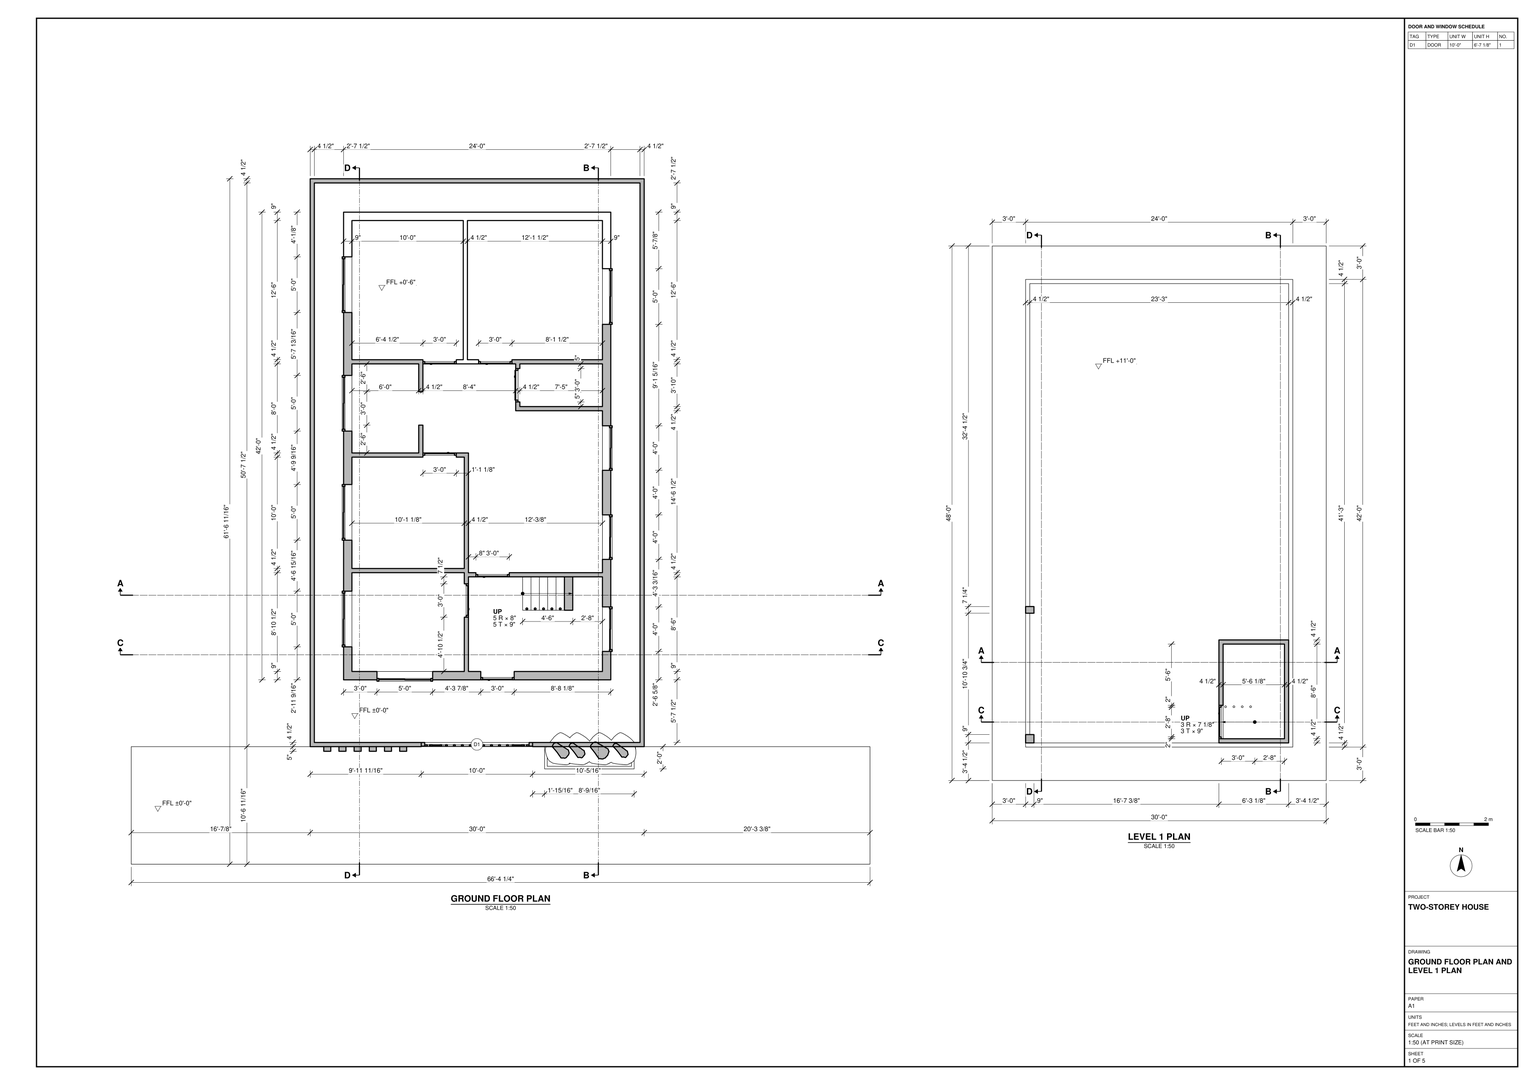
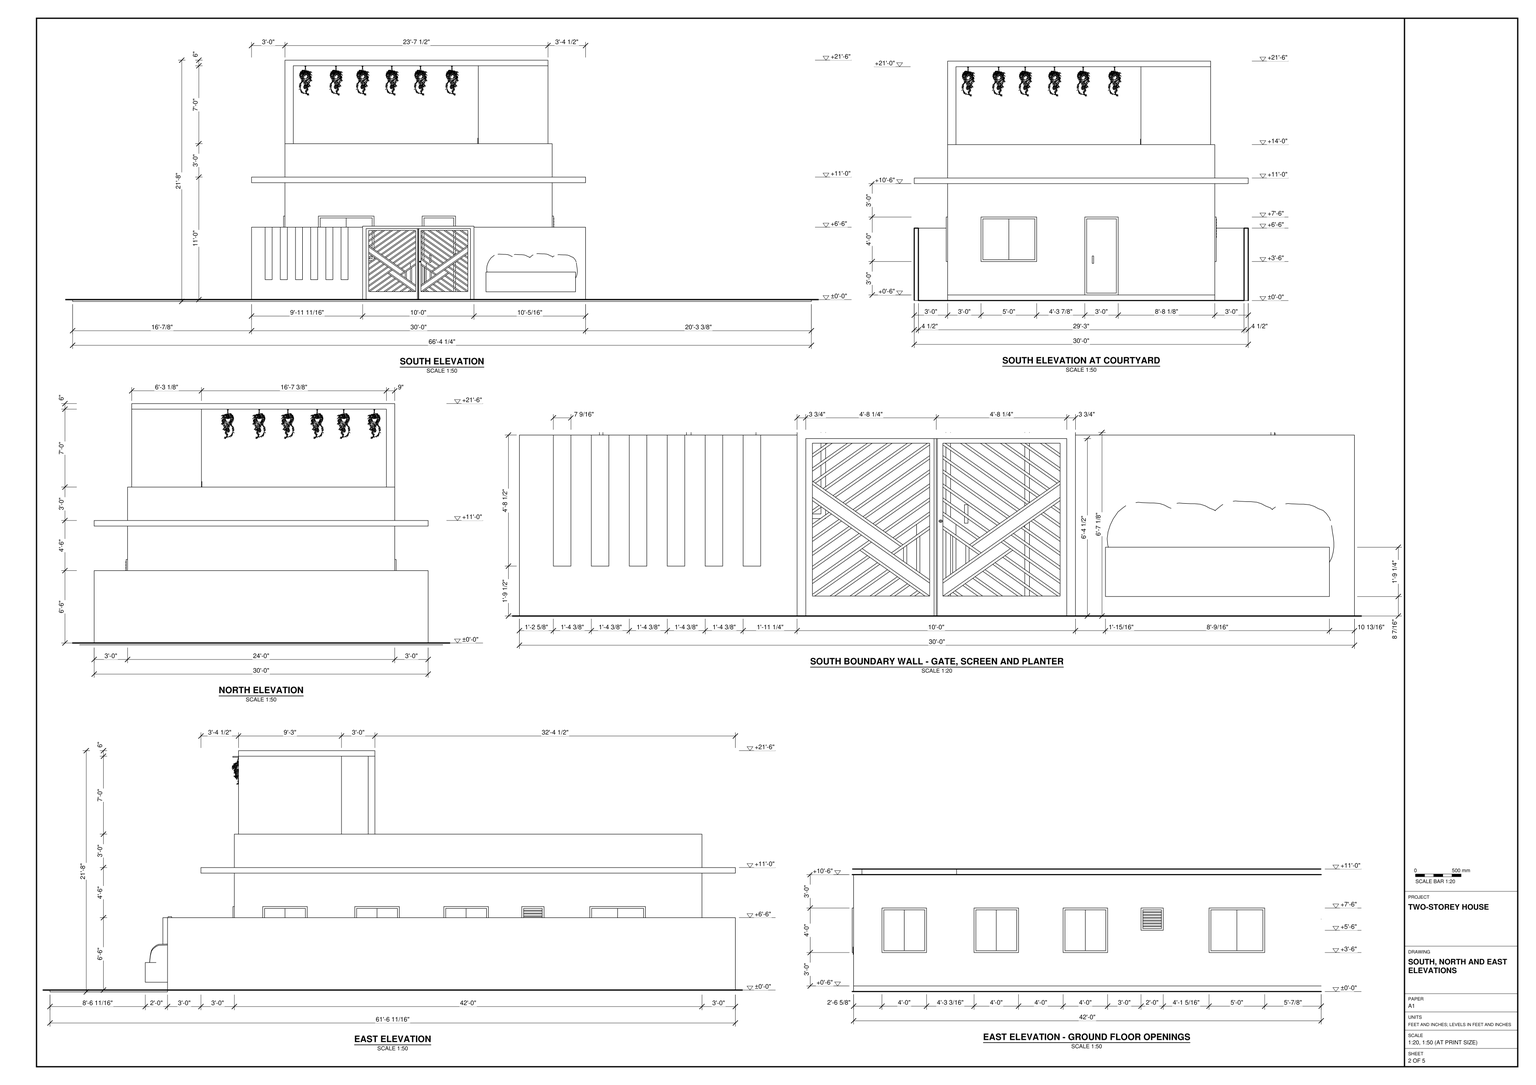
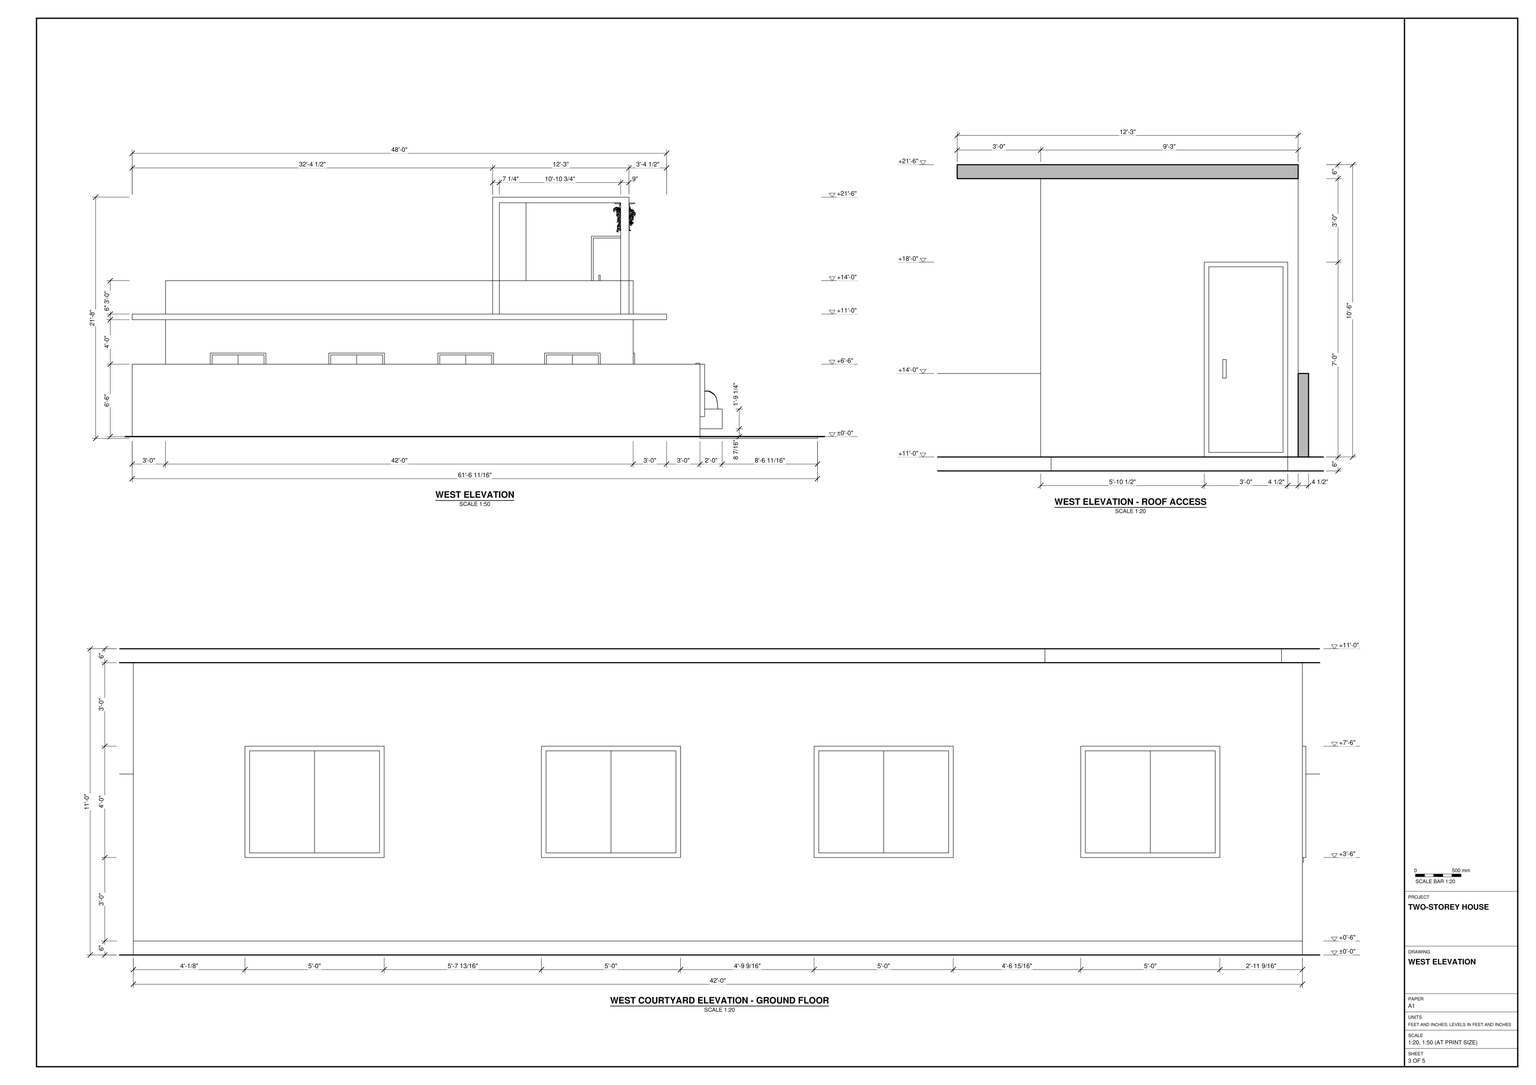
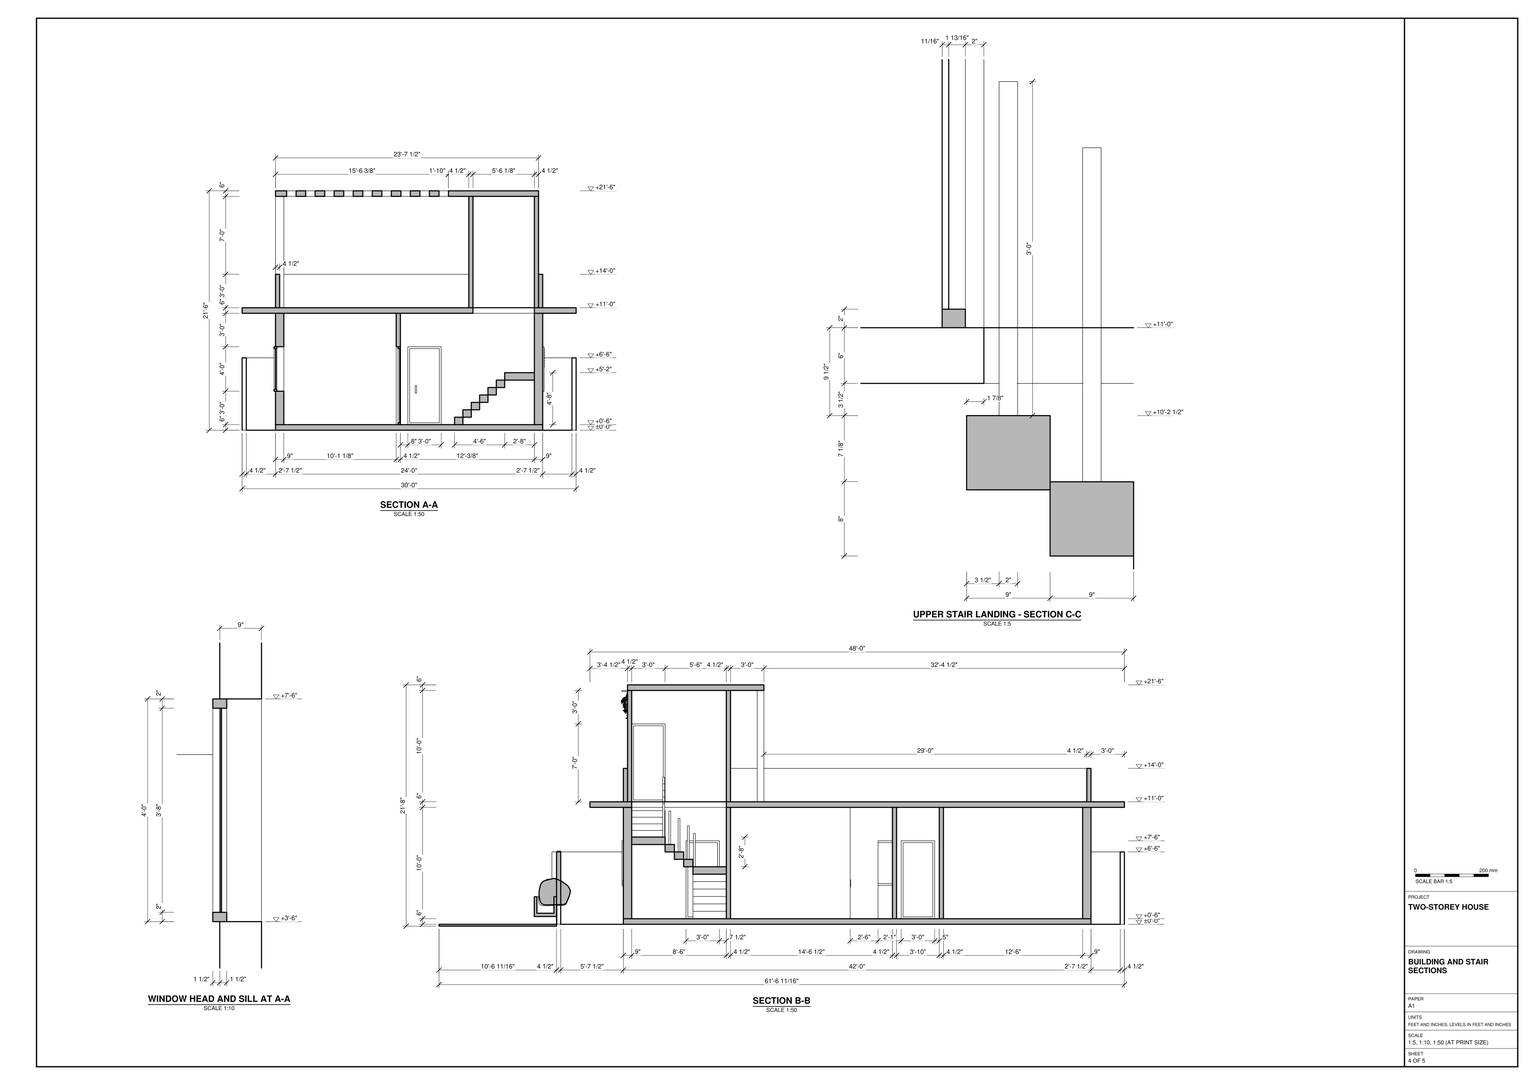
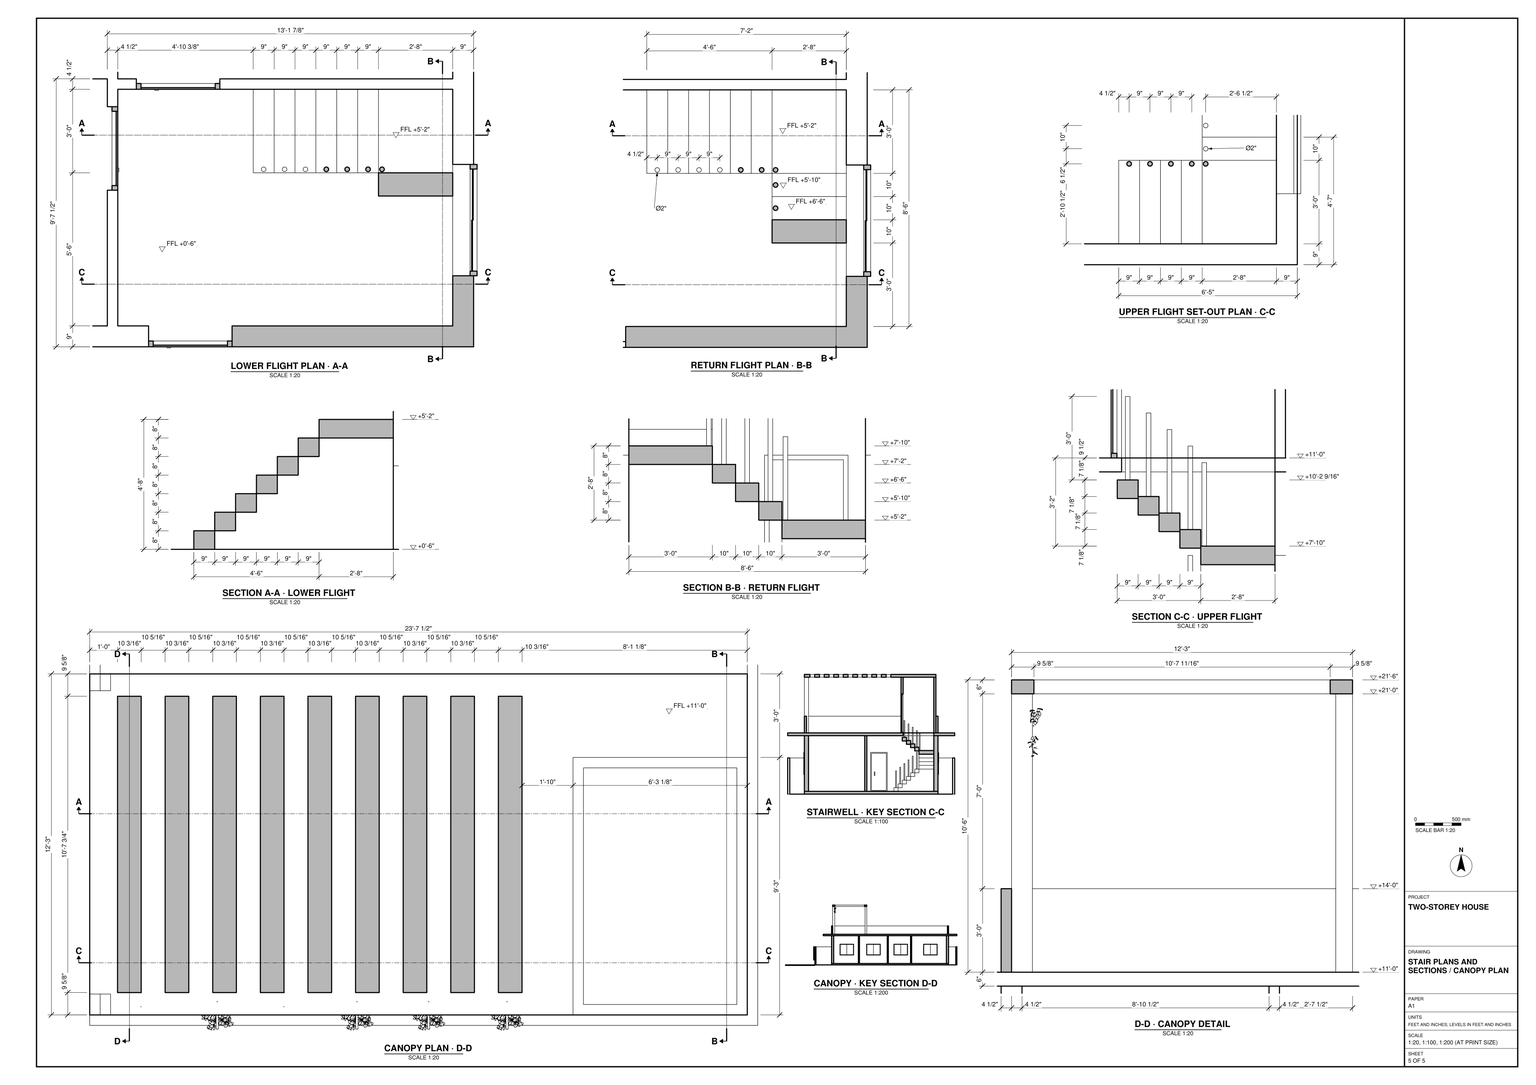
Build the house and its enclosed courtyard in SketchUp using task_files/diagram_01.pdf. Work in feet and inches. Including the ground strip outside the south boundary, the overall model extents are 66'-4 1/4" east to west, 61'-6 11/16" north to south and 21'-8" vertically. Use ±0'-0" as the ground datum and +11'-0" as the roof terrace level. Set the interior ground floor at +0'-6" as shown.

Lay out the rectangular house inside the boundary walls. Use 9" exterior walls and 4 1/2" interior partitions, following the room divisions and doorway positions on the ground floor plan. Model the courtyard entrance, window units and east wall vent from the elevations. At the south boundary, place the double gate between the slotted screen and the projecting planter.

Build the floor slabs and the stair at the southeast end of the house. Show how the stair reaches the roof access enclosure and opens onto the terrace. Distinguish the projecting terrace slab, the parapet set back from its edge and the higher flat roof over the access area. Decor and loose items, including the plants at the planter and beneath the upper roof, may be any suitable library components.

Keep walls, slabs, stairs and roofs in separate groups or components, and do the same for each furniture or joinery piece shown. Use components for repeated parts. Save one SketchUp model as output_files/two_storey_house_with_a_courtyard_and_roof_terrace.skp.

# SketchUp Ruby script. Lengths in inches.
U = 1.inch
M = Sketchup.active_model
def pt(a) = Geom::Point3d.new(a.map { |v| v * U })
def face(e, loops, mat)
  f = e.add_face(loops[0].map { |a| pt(a) })
  loops[1..].each { |l| e.add_face(l.map { |a| pt(a) }).erase! }
  f.material = f.back_material = mat if mat
  f
end
# faces: each face lists its corners as indices into pts; further lists are holes
def faces(e, pts, list, mat = nil) = list.each { |f| face(e, (f[0].is_a?(Array) ? f : [f]).map { |l| l.map { |i| pts[i] } }, mat) }
# xy, xz, yz: faces in a plane at the given z, y or x. An outline is a flat list of corners, or four numbers for a rectangle; further outlines are holes
def ring(l) = l.size == 4 ? [[l[0], l[1]], [l[2], l[1]], [l[2], l[3]], [l[0], l[3]]] : l.each_slice(2).to_a
def flat(e, list, mat, &to3) = list.each { |f| face(e, (f[0].is_a?(Array) ? f : [f]).map { |l| ring(l).map { |u, v| to3.(u, v) } }, mat) }
def xy(e, z, list, mat = nil) = flat(e, list, mat) { |x, y| [x, y, z] }
def xz(e, y, list, mat = nil) = flat(e, list, mat) { |x, z| [x, y, z] }
def yz(e, x, list, mat = nil) = flat(e, list, mat) { |y, z| [x, y, z] }
def lines(e, pts, list) = list.each { |a, b| e.add_line(pt(pts[a]), pt(pts[b])) }
# prism: a flat outline (further loops are holes) pulled along v
def prism(e, loops, v, mat = nil)
  f = face(e, loops, mat); d = Geom::Vector3d.new(v.map { |x| x * U })
  f.pushpull(f.normal.samedirection?(d) ? d.length : -d.length)
end
def box(e, o, s, mat = nil) = prism(e, [[o, [o[0] + s[0], o[1], o[2]], [o[0] + s[0], o[1] + s[1], o[2]], [o[0], o[1] + s[1], o[2]]]], [0, 0, s[2]], mat)
def at(x, y, z, deg = 0) = Geom::Transformation.translation(pt([x, y, z])) * Geom::Transformation.rotation(ORIGIN, Z_AXIS, deg.degrees)
def axes(o, x, y, z) = Geom::Transformation.new([*x, 0, *y, 0, *z, 0, *pt(o).to_a, 1])
def part(name) = M.definitions.add(name)
# library, detail: a bought-in or finely detailed component or shape, given as its bounding box
def library(name, o, s) = part(name).tap { |d| box(d.entities, o, s) }
def detail(e, o, s) = box(e.add_group.entities, o, s)
def put(e, d, t, mat = nil) = e.add_instance(d, t).tap { |i| i.material = mat if mat }
def group(e, t, mat = nil) = e.add_group.tap { |g| g.transformation = t; g.material = mat if mat }.entities
root = M.entities
M.materials.add("Asphalt A02 100cm").color = [81, 81, 83]
M.materials.add("Cementine Hexagonal Tiles 255cm").color = [92, 92, 95]
M.materials.add("Flooring Parquet Parallel E01 120cm").color = [119, 88, 63]
M.materials.add("Glass Clear 001").color = [0, 0, 0]
M.materials["Glass Clear 001"].alpha = 0.1
M.materials.add("Marble Emperador Dark 150cm").color = [81, 67, 62]
M.materials.add("Marble White SSS 100cm").color = [222, 222, 222]
M.materials.add("Metal Sandblasted Black 200cm").color = [86, 90, 95]
M.materials.add("Porcelain A02 Orange 10cm").color = [209, 126, 69]
M.materials.add("Porcelain C01 20cm").color = [125, 165, 163]
M.materials.add("Two Color Maple Panels 300cm").color = [56, 46, 41]
M.materials.add("Venetian Plaster Shadow 300cm").color = [61, 58, 77]
c1 = library("Skimmia japonica Rubella 004",[-17.08,-16.64,-0.26],[33.2,34.59,28.81])
c2 = library("Hanging Plant 111-02",[-6.97,-7.06,-31.95],[13.94,14.12,31.95])
c3 = library("gate 175k",[0,0,0],[125.98,4.13,118.11])
c4 = part("Group\#3")
box(c4.entities,[0,0,0],[28,0.31,44])
c5 = part("Group\#5")
box(c5.entities,[0,0,0],[0.31,28,44])
c6 = part("Group\#7")
box(c6.entities,[0,0,0],[0.31,28,44])
c7 = part("Group\#9")
box(c7.entities,[0,0,0],[0.31,28,44])
c8 = part("Group\#11")
box(c8.entities,[0,0,0],[0.31,28,44])
c9 = part("Group\#13")
box(c9.entities,[-0.31,0,0],[0.31,28,44])
c10 = library("Group\#14",[-1.5,0,0],[3.31,24,24])
c11 = part("Group\#17")
box(c11.entities,[-0.31,0,0],[0.31,22,44])
c12 = part("Group\#19")
box(c12.entities,[-0.31,0,0],[0.31,22,44])
c13 = part("Group\#21")
box(c13.entities,[-0.31,0,0],[0.31,22,44])
c14 = library("Group\#46",[0,0,0],[9,36,44])
c15 = library("Group\#49",[0,0,0],[9,36,44])
c16 = library("Group\#51",[0,0,0],[9,36,44])
c17 = library("Group\#53",[0,0,0],[9,36,44])
c18 = library("Group\#55",[0,0,0],[9,36,44])
c19 = library("Group\#57",[0,0,0],[9,36,44])
c20 = library("Group\#45",[0,0,0],[32,36,44])
c21 = library("Group\#48",[0,0,0],[32,10,44])
c22 = library("Group\#62",[0,0,0],[32,10,44])
c23 = library("Group\#64",[0,-2.5,0],[32,12.5,52])
c24 = library("Group\#59",[0,0,0],[9,36,44])
c25 = library("Group\#68",[0,0,0],[9,36,44])
c26 = library("Group\#70",[0,0,0],[9,36,44])
c27 = library("Group\#72",[0,0,0],[9,36,44])
c28 = library("Group\#75",[-0.5,0,0],[75.64,111,120])
put(root,c1,at(463.34,123.86,14.48))
put(root,c1,at(480.94,123.86,14.16))
put(root,c1,at(505.1875,123.86,15.05))
put(root,c1,at(527.875,123.86,13.94))
put(root,c2,at(251.0625,212.83,246))
put(root,c2,at(284.01,203.1875,246))
put(root,c2,at(312.64,212.83,246))
put(root,c2,at(344.21,203.1875,246))
put(root,c2,at(375.125,203.1875,246))
put(root,c2,at(408.96,203.1875,246))
put(root,c3,axes([312.59,127.05,-6],[0.9525,0,0],[0,1,0],[0,0,0.67]))
g1 = group(root,at(228.875,198.6875,0))
xy(g1,0,[[0,0,0,504,288,504,288,0,183.875,0,183.875,9,279,9,279,111,178.6,111,178.6,115.5,279,115.5,279,290,185.5,290,185.5,299.5,190,299.5,190,294.5,279,294.5,279,340.5,190,340.5,190,335.5,185.5,335.5,185.5,340.5,181.5,340.5,181.5,345,279,345,279,495,133.5,495,133.5,345,145.5,345,145.5,340.5,121.5,340.5,121.5,345,129,345,129,495,9,495,9,345,85.5,345,85.5,310.5,81,310.5,81,340.5,9,340.5,9,244.5,81,244.5,81,274.5,85.5,274.5,85.5,240,9,240,9,120,130.1,120,130.1,240,121.5,240,121.5,244.5,134.6,244.5,134.6,115.5,142.6,115.5,142.6,111,134.6,111,134.6,103.5,130.1,103.5,130.1,115.5,9,115.5,9,9,130.1,9,130.1,67.5,134.6,67.5,134.6,9,147.875,9,147.875,0]],"Venetian Plaster Shadow 300cm")
xy(g1,36,[[36,0,96,9],[279,30.61,288,78.61],[0,35.5625,9,95.5625],[279,129.8,288,177.8],[0,150.5,9,210.5],
  [279,225.8,288,273.8],[0,268.0625,9,328.0625],[279,383.11,288,443.11],[0,395.875,9,455.875]])
xy(g1,60,[[279,309.8,288,333.8]])
xy(g1,84,[[36,0,96,9],[147.875,0,183.875,9],[279,30.61,288,78.61],[0,35.5625,9,95.5625],[130.1,67.5,134.6,103.5],
  [142.6,111,178.6,115.5],[279,129.8,288,177.8],[0,150.5,9,210.5],[279,225.8,288,273.8],[85.5,240,121.5,244.5],
  [0,268.0625,9,328.0625],[81,274.5,85.5,310.5],[185.5,299.5,190,335.5],[279,309.8,288,333.8],[85.5,340.5,121.5,345],
  [145.5,340.5,181.5,345],[279,383.11,288,443.11],[0,395.875,9,455.875]])
xy(g1,120,[[[0,0,288,504],[134.6,115.5,134.6,244.5,85.5,244.5,85.5,340.5,185.5,340.5,185.5,290,279,290,279,115.5],[133.5,345,279,495],[9,345,129,495],[134.6,9,279,111],[9,120,130.1,240],[9,9,130.1,115.5],[9,244.5,81,340.5],[190,294.5,279,340.5]]])
xz(g1,0,[[[0,0,147.875,0,147.875,84,183.875,84,183.875,0,288,0,288,120,0,120],[36,36,96,84]]],"Porcelain C01 20cm")
xz(g1,9,[[[9,0,130.1,120],[36,36,96,84]],[134.6,0,134.6,120,279,120,279,0,183.875,0,183.875,84,147.875,84,147.875,0]],"Venetian Plaster Shadow 300cm")
xz(g1,30.61,[[279,36,288,84]])
xz(g1,35.5625,[[0,36,9,84]])
xz(g1,67.5,[[130.1,0,134.6,84]])
xz(g1,78.61,[[279,36,288,84]])
xz(g1,95.5625,[[0,36,9,84]])
xz(g1,103.5,[[130.1,0,134.6,84]])
xz(g1,111,[[134.6,0,142.6,0,142.6,84,178.6,84,178.6,0,279,0,279,120,134.6,120]],"Venetian Plaster Shadow 300cm")
xz(g1,115.5,[[9,0,130.1,120],[134.6,0,134.6,120,279,120,279,0,178.6,0,178.6,84,142.6,84,142.6,0]],"Venetian Plaster Shadow 300cm")
xz(g1,120,[[9,0,130.1,120]],"Venetian Plaster Shadow 300cm")
xz(g1,129.8,[[279,36,288,84]])
xz(g1,150.5,[[0,36,9,84]])
xz(g1,177.8,[[279,36,288,84]])
xz(g1,210.5,[[0,36,9,84]])
xz(g1,225.8,[[279,36,288,84]])
xz(g1,240,[[9,0,85.5,0,85.5,84,121.5,84,121.5,0,130.1,0,130.1,120,9,120]],"Venetian Plaster Shadow 300cm")
xz(g1,244.5,[[9,0,81,120],[121.5,0,121.5,84,85.5,84,85.5,120,134.6,120,134.6,0]],"Venetian Plaster Shadow 300cm")
xz(g1,268.0625,[[0,36,9,84]])
xz(g1,273.8,[[279,36,288,84]])
xz(g1,274.5,[[81,0,85.5,84]])
xz(g1,290,[[185.5,0,279,120]],"Venetian Plaster Shadow 300cm")
xz(g1,294.5,[[190,0,279,120]],"Venetian Plaster Shadow 300cm")
xz(g1,299.5,[[185.5,0,190,84]])
xz(g1,309.8,[[279,60,288,84]])
xz(g1,310.5,[[81,0,85.5,84]])
xz(g1,328.0625,[[0,36,9,84]])
xz(g1,333.8,[[279,60,288,84]])
xz(g1,335.5,[[185.5,0,190,84]])
xz(g1,340.5,[[9,0,81,120],[121.5,0,145.5,0,145.5,84,181.5,84,181.5,0,185.5,0,185.5,120,85.5,120,85.5,84,121.5,84],[190,0,279,120]],"Venetian Plaster Shadow 300cm")
xz(g1,345,[[9,0,9,120,129,120,129,0,121.5,0,121.5,84,85.5,84,85.5,0],[133.5,0,133.5,120,279,120,279,0,181.5,0,181.5,84,145.5,84,145.5,0]],"Venetian Plaster Shadow 300cm")
xz(g1,383.11,[[279,36,288,84]])
xz(g1,395.875,[[0,36,9,84]])
xz(g1,443.11,[[279,36,288,84]])
xz(g1,455.875,[[0,36,9,84]])
xz(g1,495,[[9,0,129,120],[133.5,0,279,120]],"Venetian Plaster Shadow 300cm")
xz(g1,504,[[0,0,288,120]],"Porcelain C01 20cm")
yz(g1,0,[[[0,0,504,120],[395.875,36,455.875,84],[268.0625,36,328.0625,84],[150.5,36,210.5,84],[35.5625,36,95.5625,84]]],"Porcelain C01 20cm")
yz(g1,9,[[[9,0,115.5,120],[35.5625,36,95.5625,84]],[[120,0,240,120],[150.5,36,210.5,84]],[[244.5,0,340.5,120],[268.0625,36,328.0625,84]],[[345,0,495,120],[395.875,36,455.875,84]]],"Venetian Plaster Shadow 300cm")
yz(g1,36,[[0,36,9,84]])
yz(g1,81,[[244.5,0,244.5,120,340.5,120,340.5,0,310.5,0,310.5,84,274.5,84,274.5,0]],"Venetian Plaster Shadow 300cm")
yz(g1,85.5,[[240,0,274.5,0,274.5,84,310.5,84,310.5,0,345,0,345,84,340.5,84,340.5,120,244.5,120,244.5,84,240,84]],"Venetian Plaster Shadow 300cm")
yz(g1,96,[[0,36,9,84]])
yz(g1,121.5,[[240,0,244.5,84],[340.5,0,345,84]])
yz(g1,129,[[345,0,495,120]],"Venetian Plaster Shadow 300cm")
yz(g1,130.1,[[9,0,9,120,115.5,120,115.5,0,103.5,0,103.5,84,67.5,84,67.5,0],[120,0,240,120]],"Venetian Plaster Shadow 300cm")
yz(g1,133.5,[[345,0,495,120]],"Venetian Plaster Shadow 300cm")
yz(g1,134.6,[[9,0,67.5,0,67.5,84,103.5,84,103.5,0,111,0,111,120,9,120],[115.5,0,244.5,120]],"Venetian Plaster Shadow 300cm")
yz(g1,142.6,[[111,0,115.5,84]])
yz(g1,145.5,[[340.5,0,345,84]])
yz(g1,147.875,[[0,0,9,84]])
yz(g1,178.6,[[111,0,115.5,84]])
yz(g1,181.5,[[340.5,0,345,84]])
yz(g1,183.875,[[0,0,9,84]])
yz(g1,185.5,[[290,0,290,120,340.5,120,340.5,0,335.5,0,335.5,84,299.5,84,299.5,0]],"Venetian Plaster Shadow 300cm")
yz(g1,190,[[294.5,0,299.5,0,299.5,84,335.5,84,335.5,0,340.5,0,340.5,120,294.5,120]],"Venetian Plaster Shadow 300cm")
yz(g1,279,[[[9,0,111,120],[30.61,36,78.61,84]]])
yz(g1,279,[[[115.5,0,290,120],[225.8,36,273.8,84],[129.8,36,177.8,84]],[[294.5,0,340.5,120],[309.8,60,333.8,84]],[[345,0,495,120],[383.11,36,443.11,84]]],"Venetian Plaster Shadow 300cm")
yz(g1,288,[[[0,0,504,120],[383.11,36,443.11,84],[225.8,36,273.8,84],[30.61,36,78.61,84],[129.8,36,177.8,84],[309.8,60,333.8,84]]],"Porcelain C01 20cm")
g2 = group(g1,at(36,0,36))
prism(g2,[[[0,-1.5,0],[60,-1.5,0],[60,-1.5,48],[0,-1.5,48]],[[58,-1.5,2],[2,-1.5,2],[2,-1.5,46],[58,-1.5,46]]],[0,3,0],"Metal Sandblasted Black 200cm")
put(g2,c4,at(2,0.25,2),"Glass Clear 001")
put(g2,c4,at(30,-0.06,2),"Glass Clear 001")
g3 = group(g1,at(0,35.5625,36))
prism(g3,[[[-1.5,0,0],[-1.5,0,48],[-1.5,60,48],[-1.5,60,0]],[[-1.5,2,2],[-1.5,58,2],[-1.5,58,46],[-1.5,2,46]]],[3,0,0],"Metal Sandblasted Black 200cm")
put(g3,c5,at(0.0625,30,2),"Glass Clear 001")
put(g3,c5,at(-0.25,2,2),"Glass Clear 001")
g4 = group(g1,at(0,150.5,36))
prism(g4,[[[-1.5,0,0],[-1.5,0,48],[-1.5,60,48],[-1.5,60,0]],[[-1.5,58,46],[-1.5,2,46],[-1.5,2,2],[-1.5,58,2]]],[3,0,0],"Metal Sandblasted Black 200cm")
put(g4,c6,at(0,30,2),"Glass Clear 001")
put(g4,c6,at(-0.31,2,2),"Glass Clear 001")
g5 = group(g1,at(0,268.0625,36))
prism(g5,[[[-1.5,60,0],[-1.5,0,0],[-1.5,0,48],[-1.5,60,48]],[[-1.5,2,46],[-1.5,2,2],[-1.5,58,2],[-1.5,58,46]]],[3,0,0],"Metal Sandblasted Black 200cm")
put(g5,c7,at(0.0625,30,2),"Glass Clear 001")
put(g5,c7,at(-0.25,2,2),"Glass Clear 001")
g6 = group(g1,at(0,395.875,36))
xy(g6,0,[[-1.5,0,1.5,60]])
xy(g6,2,[[-1.5,2,1.5,58]])
xy(g6,46,[[-1.5,2,1.5,58]])
xy(g6,48,[[-1.5,0,1.5,60]])
xz(g6,0,[[-1.5,0,1.5,48]])
xz(g6,2,[[-1.5,2,1.5,46]])
xz(g6,58,[[-1.5,2,1.5,46]])
xz(g6,60,[[-1.5,0,1.5,48]])
yz(g6,-1.5,[[[0,0,60,48],[2,2,58,46]]],"Metal Sandblasted Black 200cm")
yz(g6,1.5,[[[0,0,60,48],[2,2,58,46]]])
put(g6,c8,at(-0.1875,30,2),"Glass Clear 001")
put(g6,c8,at(-0.5,2,2),"Glass Clear 001")
g7 = group(g1,at(288,383.11,36))
prism(g7,[[[1.5,0,0],[1.5,60,0],[1.5,60,48],[1.5,0,48]],[[1.5,58,46],[1.5,58,2],[1.5,2,2],[1.5,2,46]]],[-3,0,0],"Metal Sandblasted Black 200cm")
put(g7,c9,at(-0.25,2,2),"Glass Clear 001")
put(g7,c9,at(0.06,30,2),"Glass Clear 001")
put(g1,c10,at(288,309.8,60))
g8 = group(g1,at(288,225.8,36))
prism(g8,[[[1.5,0,0],[1.5,48,0],[1.5,48,48],[1.5,0,48]],[[1.5,46,46],[1.5,46,2],[1.5,2,2],[1.5,2,46]]],[-3,0,0],"Metal Sandblasted Black 200cm")
put(g8,c11,at(0,2,2),"Glass Clear 001")
put(g8,c11,at(0.31,24,2),"Glass Clear 001")
g9 = group(g1,at(288,129.8,36))
prism(g9,[[[1.5,48,0],[1.5,48,48],[1.5,0,48],[1.5,0,0]],[[1.5,46,46],[1.5,46,2],[1.5,2,2],[1.5,2,46]]],[-3,0,0],"Metal Sandblasted Black 200cm")
put(g9,c12,at(-0.4375,2,2),"Glass Clear 001")
put(g9,c12,at(-0.12,24,2),"Glass Clear 001")
g10 = group(g1,at(288,30.61,36))
prism(g10,[[[1.5,48,0],[1.5,48,48],[1.5,0,48],[1.5,0,0]],[[1.5,46,46],[1.5,46,2],[1.5,2,2],[1.5,2,46]]],[-3,0,0],"Metal Sandblasted Black 200cm")
put(g10,c13,at(-0.5,2,2),"Glass Clear 001")
put(g10,c13,at(-0.19,24,2),"Glass Clear 001")
g11 = group(g1,at(147.875,0,0))
prism(g11,[[[36,0,0],[36,0,84],[0,0,84],[0,0,0]],[[34,0,82],[34,0,2],[2,0,2],[2,0,82]]],[0,2.5,0],"Metal Sandblasted Black 200cm")
g12 = group(g11,at(2,0,2))
box(g12,[0,0,0],[32,0.71,80],"Two Color Maple Panels 300cm")
g13 = group(g12,at(6,0,32),"Metal Sandblasted Black 200cm")
box(g13,[0,-0.5,0],[1.5,0.5,8])
g14 = group(g1,at(134.6,67.5,0))
prism(g14,[[[0,36,0],[0,36,84],[0,0,84],[0,0,0]],[[0,2,82],[0,34,82],[0,34,2],[0,2,2]]],[-2.5,0,0],"Metal Sandblasted Black 200cm")
g15 = group(g14,at(0,2,2))
xy(g15,0,[[-0.71,0,0,32]])
xy(g15,80,[[-0.71,0,0,32]])
xz(g15,0,[[-0.71,0,0,80]])
xz(g15,32,[[-0.71,0,0,80]])
yz(g15,-0.71,[[0,0,32,80]],"Two Color Maple Panels 300cm")
yz(g15,0,[[0,0,32,80]],"Two Color Maple Panels 300cm")
g16 = group(g15,at(0,6,32),"Metal Sandblasted Black 200cm")
box(g16,[0,0,0],[0.5,1.5,8])
g17 = group(g1,at(142.6,111,0))
prism(g17,[[[0,0,0],[36,0,0],[36,0,84],[0,0,84]],[[34,0,82],[34,0,2],[2,0,2],[2,0,82]]],[0,2.5,0],"Metal Sandblasted Black 200cm")
g18 = group(g17,at(2,0,2))
box(g18,[0,0,0],[32,0.71,80],"Two Color Maple Panels 300cm")
g19 = group(g18,at(6,0,32),"Metal Sandblasted Black 200cm")
box(g19,[0,-0.5,0],[1.5,0.5,8])
g20 = group(g1,at(145.5,340.5,0))
prism(g20,[[[0,0,0],[36,0,0],[36,0,84],[0,0,84]],[[2,0,82],[34,0,82],[34,0,2],[2,0,2]]],[0,2.5,0],"Metal Sandblasted Black 200cm")
g21 = group(g20,at(2,0,2))
box(g21,[0,0,0],[32,0.71,80],"Two Color Maple Panels 300cm")
g22 = group(g21,at(6,0,32),"Metal Sandblasted Black 200cm")
box(g22,[0,-0.5,0],[1.5,0.5,8])
g23 = group(g1,at(85.5,340.5,0))
prism(g23,[[[36,0,0],[36,0,84],[0,0,84],[0,0,0]],[[34,0,82],[34,0,2],[2,0,2],[2,0,82]]],[0,2.5,0],"Metal Sandblasted Black 200cm")
g24 = group(g23,at(2,0,2))
box(g24,[0,0,0],[32,0.71,80],"Two Color Maple Panels 300cm")
g25 = group(g24,at(6,0,32),"Metal Sandblasted Black 200cm")
box(g25,[0,-0.5,0],[1.5,0.5,8])
g26 = group(g1,at(185.5,299.5,0))
prism(g26,[[[0,0,0],[0,0,84],[0,36,84],[0,36,0]],[[0,2,82],[0,2,2],[0,34,2],[0,34,82]]],[2.5,0,0],"Metal Sandblasted Black 200cm")
g27 = group(g26,at(0,2,2))
box(g27,[-0.71,0,0],[0.71,32,80],"Two Color Maple Panels 300cm")
g28 = group(g27,at(-0.71,26,32),"Metal Sandblasted Black 200cm")
box(g28,[-0.5,-1.5,0],[0.5,1.5,8])
g29 = group(g1,at(85.5,244.5,0))
prism(g29,[[[36,0,84],[36,0,0],[0,0,0],[0,0,84]],[[2,0,82],[2,0,2],[34,0,2],[34,0,82]]],[0,-2.5,0],"Metal Sandblasted Black 200cm")
g30 = group(g29,at(2,0,2))
box(g30,[0,-0.71,0],[32,0.71,80],"Two Color Maple Panels 300cm")
g31 = group(g30,at(26,0,32),"Metal Sandblasted Black 200cm")
box(g31,[-1.5,0,0],[1.5,0.5,8])
g32 = group(root,at(228.875,198.6875,-6))
box(g32,[0,0,0],[288,504,6],"Marble White SSS 100cm")
put(root,c14,at(421.875,273.6875,0))
put(root,c15,at(430.875,273.6875,8))
put(root,c16,at(439.875,273.6875,16))
put(root,c17,at(448.875,273.6875,24))
put(root,c18,at(457.875,273.6875,32))
put(root,c19,at(466.875,273.6875,40))
put(root,c20,at(475.875,273.6875,48))
put(root,c21,at(475.875,263.6875,56))
put(root,c22,at(475.875,253.6875,64))
put(root,c23,at(475.875,243.6875,72))
g33 = group(root,at(475.875,233.6875,80))
box(g33,[0,-26,0],[32,36,8],"Marble White SSS 100cm")
put(root,c24,at(466.875,207.6875,87.13))
put(root,c25,at(457.875,207.6875,94.26))
put(root,c26,at(448.875,207.6875,101.4))
put(root,c27,at(439.875,207.6875,108.53))
g34 = group(root,at(192.875,126.6875,-6))
xy(g34,0,[[4.5,4.5,355.5,607.5]],"Cementine Hexagonal Tiles 255cm")
xy(g34,78,[[0,0,119.71,0,119.71,4.5,4.5,4.5,4.5,607.5,355.5,607.5,355.5,4.5,239.71,4.5,239.71,0,360,0,360,612,0,612]])
xz(g34,0,[[0,0,119.71,78],[239.71,0,360,78]],"Porcelain A02 Orange 10cm")
xz(g34,4.5,[[4.5,0,119.71,78],[239.71,0,355.5,78]])
xz(g34,607.5,[[4.5,0,355.5,78]])
xz(g34,612,[[0,0,360,78]],"Porcelain A02 Orange 10cm")
yz(g34,0,[[0,0,612,78]],"Porcelain A02 Orange 10cm")
yz(g34,4.5,[[4.5,0,607.5,78]])
yz(g34,119.71,[[0,0,4.5,78]])
yz(g34,239.71,[[0,0,4.5,78]])
yz(g34,355.5,[[4.5,0,607.5,78]])
yz(g34,360,[[0,0,612,78]],"Porcelain A02 Orange 10cm")
p = [[119.71,0,0],[239.71,0,0]]
lines(g34,p,[[0,1]])
g35 = group(g34,at(14.63,0,21.5),"Flooring Parquet Parallel E01 120cm")
box(g35,[0,-5,0],[7.5625,5,56.5],"Flooring Parquet Parallel E01 120cm")
g36 = group(g34,at(31,0,21.5),"Flooring Parquet Parallel E01 120cm")
box(g36,[0,-5,0],[7.5625,5,56.5],"Flooring Parquet Parallel E01 120cm")
g37 = group(g34,at(47.36,0,21.5),"Flooring Parquet Parallel E01 120cm")
box(g37,[0,-5,0],[7.5625,5,56.5],"Flooring Parquet Parallel E01 120cm")
g38 = group(g34,at(63.72,0,21.5),"Flooring Parquet Parallel E01 120cm")
box(g38,[0,-5,0],[7.5625,5,56.5],"Flooring Parquet Parallel E01 120cm")
g39 = group(g34,at(80.08,0,21.5),"Flooring Parquet Parallel E01 120cm")
box(g39,[0,-5,0],[7.5625,5,56.5],"Flooring Parquet Parallel E01 120cm")
g40 = group(g34,at(96.45,0,21.5),"Flooring Parquet Parallel E01 120cm")
box(g40,[0,-5,0],[7.5625,5,56.5],"Flooring Parquet Parallel E01 120cm")
g41 = group(g34,at(252.65,0,8.41),"Flooring Parquet Parallel E01 120cm")
xy(g41,0,[[0,-24,96.5625,0]],"Flooring Parquet Parallel E01 120cm")
xy(g41,3.5,[[2.83,-21.17,93.74,-2.83]],"Flooring Parquet Parallel E01 120cm")
xy(g41,21.25,[[[0,-24,96.5625,0],[2.83,-21.17,93.74,-2.83]]],"Flooring Parquet Parallel E01 120cm")
xz(g41,-24,[[0,0,96.5625,21.25]],"Flooring Parquet Parallel E01 120cm")
xz(g41,-21.17,[[2.83,3.5,93.74,21.25]],"Flooring Parquet Parallel E01 120cm")
xz(g41,-2.83,[[2.83,3.5,93.74,21.25]],"Flooring Parquet Parallel E01 120cm")
xz(g41,0,[[0,0,96.5625,21.25]],"Flooring Parquet Parallel E01 120cm")
yz(g41,0,[[-24,0,0,21.25]],"Flooring Parquet Parallel E01 120cm")
yz(g41,2.83,[[-21.17,3.5,-2.83,21.25]],"Flooring Parquet Parallel E01 120cm")
yz(g41,93.74,[[-21.17,3.5,-2.83,21.25]],"Flooring Parquet Parallel E01 120cm")
yz(g41,96.5625,[[-24,0,0,21.25]],"Flooring Parquet Parallel E01 120cm")
g42 = group(root,at(192.875,162.6875,120))
g43 = group(g42,at(36,36,0))
prism(g43,[[[-36,-36,0],[-36,540,0],[324,540,0],[324,-36,0]],[[212.86,111,0],[212.86,9,0],[279,9,0],[279,111,0]]],[0,0,6],"Marble Emperador Dark 150cm")
put(g43,c28,at(208.36,4.5,6),"Porcelain C01 20cm")
g44 = group(g43,at(0,0,6),"Porcelain A02 Orange 10cm")
prism(g44,[[[0,0,0],[0,504,0],[288,504,0],[288,0,0]],[[4.5,4.5,0],[283.5,4.5,0],[283.5,499.5,0],[4.5,499.5,0]]],[0,0,36],"Porcelain A02 Orange 10cm")
g45 = group(g42,at(244.36,69.42,126))
xy(g45,-120,[[-208.36,-28.92,-199.36,-19.92],[-208.36,110.85,-199.36,118.08]],"Metal Sandblasted Black 200cm")
xy(g45,0,[[[-199.36,-28.92,-199.36,-19.92,-208.36,-19.92,-208.36,110.85,-199.36,110.85,-199.36,118.08,75.14,118.08,75.14,-28.92],[-32.17,-19.28,-21.98,108.44],[-52.69,-19.28,-42.51,108.44],[-73.22,-19.28,-63.03,108.44],[-93.74,-19.28,-83.55,108.44],[-134.79,-19.28,-124.6,108.44],[-114.27,-19.28,-104.08,108.44],[-155.31,-19.28,-145.125,108.44],[-175.84,-19.28,-165.65,108.44],[-196.36,-19.28,-186.17,108.44]]],"Metal Sandblasted Black 200cm")
xy(g45,6,[[[-208.36,-28.92,75.14,118.08],[-196.36,-19.28,-186.17,108.44],[-175.84,-19.28,-165.65,108.44],[-155.31,-19.28,-145.125,108.44],[-134.79,-19.28,-124.6,108.44],[-114.27,-19.28,-104.08,108.44],[-93.74,-19.28,-83.55,108.44],[-73.22,-19.28,-63.03,108.44],[-52.69,-19.28,-42.51,108.44],[-32.17,-19.28,-21.98,108.44]]],"Metal Sandblasted Black 200cm")
xz(g45,-28.92,[[-208.36,-120,-199.36,-120,-199.36,0,75.14,0,75.14,6,-208.36,6]],"Metal Sandblasted Black 200cm")
xz(g45,-19.92,[[-208.36,-120,-199.36,0]],"Metal Sandblasted Black 200cm")
xz(g45,-19.28,[[-196.36,0,-186.17,6],[-175.84,0,-165.65,6],[-155.31,0,-145.125,6],[-134.79,0,-124.6,6],[-114.27,0,-104.08,6],
  [-93.74,0,-83.55,6],[-73.22,0,-63.03,6],[-52.69,0,-42.51,6],[-32.17,0,-21.98,6]],"Metal Sandblasted Black 200cm")
xz(g45,108.44,[[-196.36,0,-186.17,6],[-175.84,0,-165.65,6],[-155.31,0,-145.125,6],[-134.79,0,-124.6,6],[-114.27,0,-104.08,6],
  [-93.74,0,-83.55,6],[-73.22,0,-63.03,6],[-52.69,0,-42.51,6],[-32.17,0,-21.98,6]],"Metal Sandblasted Black 200cm")
xz(g45,110.85,[[-208.36,-120,-199.36,0]],"Metal Sandblasted Black 200cm")
xz(g45,118.08,[[-208.36,-120,-208.36,6,75.14,6,75.14,0,-199.36,0,-199.36,-120]],"Metal Sandblasted Black 200cm")
yz(g45,-208.36,[[-28.92,-120,-28.92,6,118.08,6,118.08,-120,110.85,-120,110.85,0,-19.92,0,-19.92,-120]],"Metal Sandblasted Black 200cm")
yz(g45,-199.36,[[-28.92,-120,-19.92,0],[110.85,-120,118.08,0]],"Metal Sandblasted Black 200cm")
yz(g45,-196.36,[[-19.28,0,108.44,6]],"Metal Sandblasted Black 200cm")
yz(g45,-186.17,[[-19.28,0,108.44,6]],"Metal Sandblasted Black 200cm")
yz(g45,-175.84,[[-19.28,0,108.44,6]],"Metal Sandblasted Black 200cm")
yz(g45,-165.65,[[-19.28,0,108.44,6]],"Metal Sandblasted Black 200cm")
yz(g45,-155.31,[[-19.28,0,108.44,6]],"Metal Sandblasted Black 200cm")
yz(g45,-145.125,[[-19.28,0,108.44,6]],"Metal Sandblasted Black 200cm")
yz(g45,-134.79,[[-19.28,0,108.44,6]],"Metal Sandblasted Black 200cm")
yz(g45,-124.6,[[-19.28,0,108.44,6]],"Metal Sandblasted Black 200cm")
yz(g45,-114.27,[[-19.28,0,108.44,6]],"Metal Sandblasted Black 200cm")
yz(g45,-104.08,[[-19.28,0,108.44,6]],"Metal Sandblasted Black 200cm")
yz(g45,-93.74,[[-19.28,0,108.44,6]],"Metal Sandblasted Black 200cm")
yz(g45,-83.55,[[-19.28,0,108.44,6]],"Metal Sandblasted Black 200cm")
yz(g45,-73.22,[[-19.28,0,108.44,6]],"Metal Sandblasted Black 200cm")
yz(g45,-63.03,[[-19.28,0,108.44,6]],"Metal Sandblasted Black 200cm")
yz(g45,-52.69,[[-19.28,0,108.44,6]],"Metal Sandblasted Black 200cm")
yz(g45,-42.51,[[-19.28,0,108.44,6]],"Metal Sandblasted Black 200cm")
yz(g45,-32.17,[[-19.28,0,108.44,6]],"Metal Sandblasted Black 200cm")
yz(g45,-21.98,[[-19.28,0,108.44,6]],"Metal Sandblasted Black 200cm")
yz(g45,75.14,[[-28.92,0,118.08,6]],"Metal Sandblasted Black 200cm")
g46 = group(root,at(192.875,0,-6),"Asphalt A02 100cm")
box(g46,[-192.875,0,-2],[796.25,126.6875,2],"Asphalt A02 100cm")
